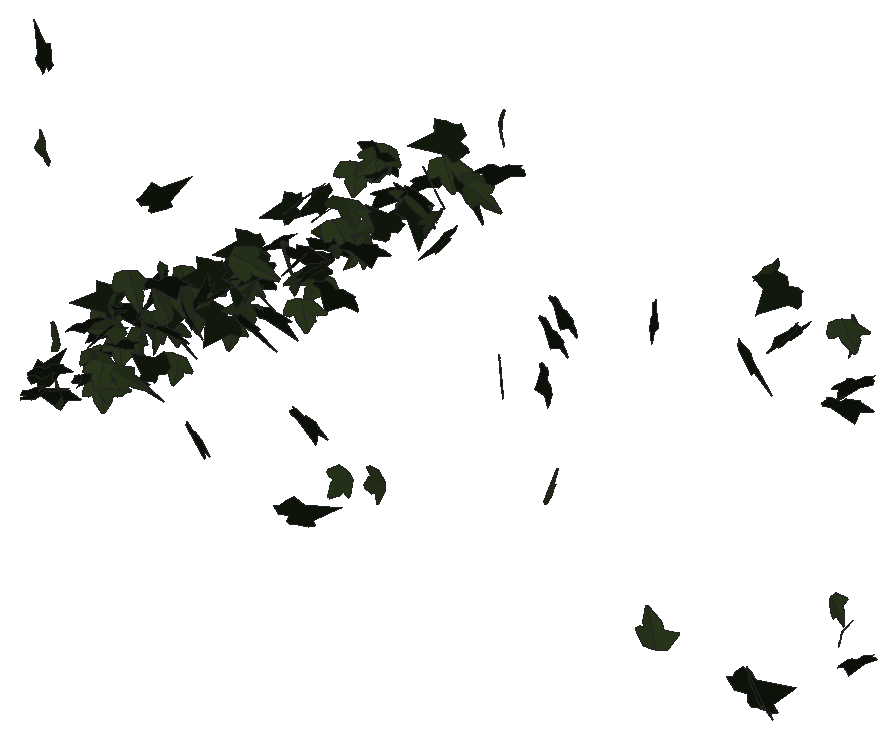
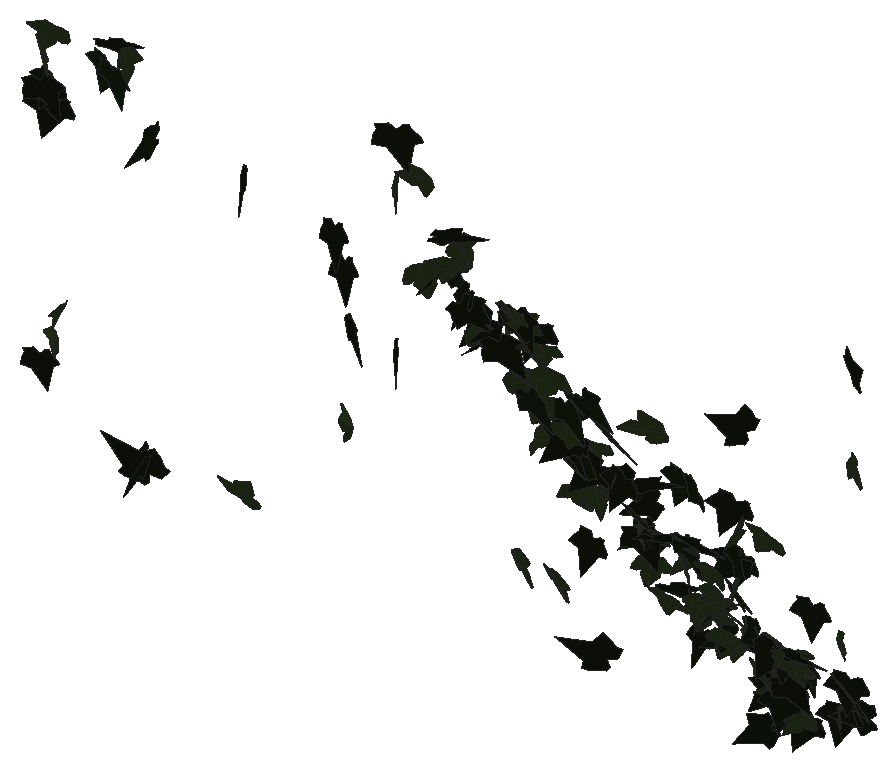
# SketchUp Ruby script. Lengths in inches.
U = 1.inch
M = Sketchup.active_model
def pt(a) = Geom::Point3d.new(a.map { |v| v * U })
def face(e, loops, mat)
  f = e.add_face(loops[0].map { |a| pt(a) })
  loops[1..].each { |l| e.add_face(l.map { |a| pt(a) }).erase! }
  f.material = f.back_material = mat if mat
  f
end
# faces: each face lists its corners as indices into pts; further lists are holes
def faces(e, pts, list, mat = nil) = list.each { |f| face(e, (f[0].is_a?(Array) ? f : [f]).map { |l| l.map { |i| pts[i] } }, mat) }
# xy, xz, yz: faces in a plane at the given z, y or x. An outline is a flat list of corners, or four numbers for a rectangle; further outlines are holes
def ring(l) = l.size == 4 ? [[l[0], l[1]], [l[2], l[1]], [l[2], l[3]], [l[0], l[3]]] : l.each_slice(2).to_a
def flat(e, list, mat, &to3) = list.each { |f| face(e, (f[0].is_a?(Array) ? f : [f]).map { |l| ring(l).map { |u, v| to3.(u, v) } }, mat) }
def xy(e, z, list, mat = nil) = flat(e, list, mat) { |x, y| [x, y, z] }
def xz(e, y, list, mat = nil) = flat(e, list, mat) { |x, z| [x, y, z] }
def yz(e, x, list, mat = nil) = flat(e, list, mat) { |y, z| [x, y, z] }
def lines(e, pts, list) = list.each { |a, b| e.add_line(pt(pts[a]), pt(pts[b])) }
# prism: a flat outline (further loops are holes) pulled along v
def prism(e, loops, v, mat = nil)
  f = face(e, loops, mat); d = Geom::Vector3d.new(v.map { |x| x * U })
  f.pushpull(f.normal.samedirection?(d) ? d.length : -d.length)
end
def box(e, o, s, mat = nil) = prism(e, [[o, [o[0] + s[0], o[1], o[2]], [o[0] + s[0], o[1] + s[1], o[2]], [o[0], o[1] + s[1], o[2]]]], [0, 0, s[2]], mat)
def at(x, y, z, deg = 0) = Geom::Transformation.translation(pt([x, y, z])) * Geom::Transformation.rotation(ORIGIN, Z_AXIS, deg.degrees)
def axes(o, x, y, z) = Geom::Transformation.new([*x, 0, *y, 0, *z, 0, *pt(o).to_a, 1])
def part(name) = M.definitions.add(name)
# library, detail: a bought-in or finely detailed component or shape, given as its bounding box
def library(name, o, s) = part(name).tap { |d| box(d.entities, o, s) }
def detail(e, o, s) = box(e.add_group.entities, o, s)
def put(e, d, t, mat = nil) = e.add_instance(d, t).tap { |i| i.material = mat if mat }
def group(e, t, mat = nil) = e.add_group.tap { |g| g.transformation = t; g.material = mat if mat }.entities
root = M.entities
M.materials.add("1026 AP 7946 SUNNY SIDE UP").color = [254, 231, 186]
M.materials.add("efeu1").color = [18, 25, 13]
M.materials.add("efeu2").color = [43, 57, 29]
c1 = part("ivyleaf_10")
p = [[0,0.5,-0.03],[-0.0625,2.02,-0.43],[-0.19,2.01,-0.46],[-0.54,1.05,-0.29],[-0.52,0.625,-0.18],[-0.83,0.76,-0.28],
  [-1.16,0.64,-0.33],[-1.15,0.33,-0.24],[-0.77,-0.39,0.02],[-0.3,-0.51,0.16],[0.04,-0.48,0.23],[-0.02,2.01,-0.4375],
  [-0.06,2.01,-0.43],[0.04,-0.49,0.23],[0.67,-0.49,0.14],[1.38,0.36,-0.2],[1.375,0.51,-0.24],[0.81,0.65,-0.19],
  [0.62,0.59,-0.15],[0.6,1.09,-0.28],[0.5,1.23,-0.31]]
faces(c1.entities,p,[[0,1,2,3,4,5,6,7,8,9,10],[11,12,0,13,14,15,16,17,18,19,20]],"efeu2")
c2 = part("ivyleaf_9")
p = [[1.54,2.16,1.25],[1.36,2.04,1.19],[-0.21,0.99,0.68],[-0.71,1.11,0.82],[-0.85,0.86,0.67],[-0.8,0.17,0.21],
  [-0.9,-0.01,0.1],[-0.67,-0.16,-0.02],[-0.08,-0.08,-0.05],[-0.03,-0.6,-0.4],[0.65,-0.88,-0.66],[0.83,-0.6,-0.49],
  [1.29,-0.42,-0.43],[1.8125,-0.07,-0.26],[1.21,0.44,0.15]]
faces(c2.entities,p,[[0,1,2,3,4,5,6,7,8,9,10,11,12,13,14]],"efeu1")
put(root,c1,axes([119.91,212.96,275.25],[-0.15786,0.09565,0.26441],[-0.34427,0.13528,-0.13967],[-0.25746,-0.23953,0.02464]),"1026 AP 7946 SUNNY SIDE UP")
put(root,c2,axes([119.46,212.93,268.7],[0.22563,0.03038,0.22502],[0.27226,0.14554,-0.1373],[-0.2143,0.21689,0.06248]),"1026 AP 7946 SUNNY SIDE UP")
put(root,c2,axes([119.64,213.11,269.07],[-0.17228,0.27616,0.11],[0.07778,-0.09348,0.30532],[0.45812,0.11972,-0.01047]),"1026 AP 7946 SUNNY SIDE UP")
put(root,c2,axes([119.96,212.91,277.56],[0.02395,-0.02649,0.33545],[-0.08757,0.32114,0.03146],[-0.50642,-0.05678,0.01042]),"1026 AP 7946 SUNNY SIDE UP")
put(root,c2,axes([119.96,212.98,269.53],[0.1913,0.22813,-0.05414],[-0.02362,-0.05296,-0.2664],[-0.36782,0.12205,-0.01105]),"1026 AP 7946 SUNNY SIDE UP")
put(root,c1,axes([120.09,213.29,268.71],[-0.01512,0.00573,-0.26968],[-0.14913,0.24412,0.01053],[0.38382,0.09508,-0.00654]),"1026 AP 7946 SUNNY SIDE UP")
put(root,c2,axes([119.97,213.21,268.81],[0.27016,0.18563,-0.0682],[-0.07693,-0.04634,-0.26081],[-0.30077,0.1786,0.00545]),"1026 AP 7946 SUNNY SIDE UP")
put(root,c1,axes([120.29,212.93,270.43],[-0.03129,-0.00435,-0.27853],[-0.17285,0.24779,0.00568],[0.38842,0.10992,-0.01991]),"1026 AP 7946 SUNNY SIDE UP")
put(root,c1,axes([120.02,214.64,269.24],[-0.20622,-0.18907,-0.13238],[0.24349,0.03403,-0.21602],[0.26314,-0.17967,0.09614]),"1026 AP 7946 SUNNY SIDE UP")
put(root,c1,axes([120.26,214.67,270.56],[0.41937,0.01395,-0.04707],[-0.06964,-0.02611,-0.27423],[-0.02847,0.26935,-0.02255]),"1026 AP 7946 SUNNY SIDE UP")
put(root,c2,axes([120.25,214.14,268.92],[0.27349,0.19928,-0.00399],[0.01534,-0.01514,-0.272],[-0.31307,0.17334,-0.01681]),"1026 AP 7946 SUNNY SIDE UP")
put(root,c2,axes([120.48,214.59,270.05],[0.01871,0.2119,-0.1617],[-0.10982,-0.15018,-0.21357],[-0.401,0.05102,0.05095]),"1026 AP 7946 SUNNY SIDE UP")
put(root,c2,axes([120.63,214.65,270.8],[-0.36738,0.02844,0.14169],[-0.21929,-0.01824,-0.24058],[-0.02385,-0.27042,0.02952]),"1026 AP 7946 SUNNY SIDE UP")
put(root,c1,axes([120.27,214.49,269.3],[-0.39403,0.07374,-0.08104],[0.10252,-0.05619,-0.26715],[-0.13563,-0.2567,0.0335]),"1026 AP 7946 SUNNY SIDE UP")
put(root,c2,axes([120.49,214.66,268.96],[-0.24093,-0.22018,0.04193],[-0.01299,-0.04524,-0.27593],[0.35221,-0.15229,0.01851]),"1026 AP 7946 SUNNY SIDE UP")
put(root,c2,axes([120.57,214.67,269.59],[0.15949,0.24453,-0.00867],[-0.00799,-0.00851,-0.27277],[-0.38472,0.10155,0.00207]),"1026 AP 7946 SUNNY SIDE UP")
put(root,c1,axes([120.8,214.41,270.27],[0.11431,0.06577,-0.26321],[-0.39441,-0.06612,-0.09131],[-0.13039,0.25765,0.04546]),"1026 AP 7946 SUNNY SIDE UP")
put(root,c1,axes([120.62,214.61,270.73],[-0.05219,0.21044,0.17672],[-0.07529,0.16435,-0.21782],[-0.41901,-0.05574,0.01713]),"1026 AP 7946 SUNNY SIDE UP")
put(root,c2,axes([120.75,214.37,270.31],[-0.17195,0.20293,-0.15062],[0.0715,-0.14205,-0.23712],[-0.3878,-0.11617,0.02307]),"1026 AP 7946 SUNNY SIDE UP")
put(root,c1,axes([120.7,213.97,268.87],[0.34189,0.14817,0.03738],[0.06074,0.00614,-0.27049],[-0.23172,0.22022,-0.01574]),"1026 AP 7946 SUNNY SIDE UP")
put(root,c1,axes([120.74,214.68,269.73],[0.32211,0.16897,-0.00307],[0.01634,-0.01878,-0.27281],[-0.26525,0.20403,-0.02054]),"1026 AP 7946 SUNNY SIDE UP")
put(root,c2,axes([120.79,214.58,269.77],[0.33822,0.14743,0.0544],[0.08034,0.01723,-0.26814],[-0.2323,0.22061,-0.01353]),"1026 AP 7946 SUNNY SIDE UP")
put(root,c2,axes([121.125,213.16,269.66],[-0.06173,0.24971,0.08639],[-0.03885,0.07948,-0.25967],[-0.41165,-0.04495,0.01155]),"1026 AP 7946 SUNNY SIDE UP")
put(root,c2,axes([120.89,214.5625,270.75],[0.32899,0.16773,-0.01701],[-0.00017,-0.02769,-0.27553],[-0.26517,0.20812,-0.02092]),"1026 AP 7946 SUNNY SIDE UP")
put(root,c2,axes([121.04,212.99,271.1],[0.10218,0.26159,0.00145],[-0.00734,0.00108,-0.27763],[-0.41125,0.06497,0.00531]),"1026 AP 7946 SUNNY SIDE UP")
put(root,c2,axes([120.8,214.875,268.82],[0.42122,-0.02405,0.03637],[0.05631,0.00262,-0.277],[0.03694,0.2702,0.00752]),"1026 AP 7946 SUNNY SIDE UP")
put(root,c1,axes([121.34,213.29,269.91],[0.35846,0.13176,-0.0463],[-0.04318,-0.04344,-0.27043],[-0.21499,0.22841,-0.02289]),"1026 AP 7946 SUNNY SIDE UP")
put(root,c1,axes([121.26,214.71,270.125],[0.31847,-0.13253,0.1168],[0.15104,-0.06165,-0.24971],[0.22982,0.22416,0.00225]),"1026 AP 7946 SUNNY SIDE UP")
put(root,c1,axes([121.31,213.47,269.3],[0.0223,-0.11422,-0.24883],[0.23509,0.20313,-0.08897],[0.34707,-0.13025,0.07625]),"1026 AP 7946 SUNNY SIDE UP")
put(root,c2,axes([121.5,214.43,270.85],[0.07705,0.0999,0.26153],[0.12751,0.24034,-0.1124],[-0.40872,0.09381,0.01424]),"1026 AP 7946 SUNNY SIDE UP")
put(root,c1,axes([121.67,214.7,270.68],[0.1666,0.25002,0.0705],[0.05344,0.05835,-0.27927],[-0.40349,0.11096,-0.00788]),"1026 AP 7946 SUNNY SIDE UP")
put(root,c1,axes([121.65,214.41,270.84],[-0.171,0.10534,-0.23901],[0.20783,-0.19309,-0.15487],[-0.34353,-0.16925,0.02528]),"1026 AP 7946 SUNNY SIDE UP")
put(root,c1,axes([121.88,214.58,270.57],[-0.01676,0.23894,-0.14875],[-0.01049,-0.14602,-0.24698],[-0.43996,-0.00562,0.01156]),"1026 AP 7946 SUNNY SIDE UP")
put(root,c1,axes([121.97,214.63,272.05],[-0.15017,0.25701,0.03144],[-0.03386,0.02297,-0.28205],[-0.40529,-0.09715,0.01191]),"1026 AP 7946 SUNNY SIDE UP")
put(root,c2,axes([122.11,214.61,271.91],[-0.33312,0.07759,-0.16813],[0.21896,-0.09123,-0.23082],[-0.18208,-0.25167,0.03003]),"1026 AP 7946 SUNNY SIDE UP")
put(root,c1,axes([121.8,213.35,269.86],[0.12396,0.00046,0.2645],[0.37022,0.10696,-0.07405],[-0.16098,0.24636,0.03337]),"1026 AP 7946 SUNNY SIDE UP")
put(root,c1,axes([122.17,214.77,270.69],[-0.42176,0.0219,-0.02374],[0.03258,-0.02942,-0.27596],[-0.03809,-0.26761,0.0268]),"1026 AP 7946 SUNNY SIDE UP")
put(root,c2,axes([122.09,214.71,270.67],[0.30629,-0.18532,0.01811],[0.03364,-0.00452,-0.27676],[0.29093,0.19563,0.01294]),"1026 AP 7946 SUNNY SIDE UP")
put(root,c2,axes([122.31,214.8,271.34],[-0.13753,-0.25693,0.08002],[-0.00879,-0.08146,-0.27931],[0.42264,-0.0853,0.02023]),"1026 AP 7946 SUNNY SIDE UP")
put(root,c1,axes([122.2,213.18,272.57],[0.44241,-0.00955,0.17236],[0.26066,-0.03276,-0.28922],[0.03918,0.32573,-0.02211]),"1026 AP 7946 SUNNY SIDE UP")
put(root,c1,axes([122.47,214.74,271.51],[0.40201,0.11508,-0.04344],[-0.05353,-0.02862,-0.28874],[-0.1855,0.25764,-0.01084]),"1026 AP 7946 SUNNY SIDE UP")
put(root,c2,axes([122.82,213.43,270.25],[-0.11045,0.18845,0.19054],[-0.22804,0.13115,-0.19478],[-0.34555,-0.14679,0.06763]),"1026 AP 7946 SUNNY SIDE UP")
put(root,c1,axes([122.54,214.7,271.67],[-0.37148,0.11771,-0.06832],[0.06243,-0.06857,-0.2688],[-0.2036,-0.23579,0.04223]),"1026 AP 7946 SUNNY SIDE UP")
put(root,c2,axes([122.64,214.67,271.32],[0.29862,-0.1524,-0.15109],[-0.20205,0.07196,-0.24951],[0.26297,0.22835,-0.02014]),"1026 AP 7946 SUNNY SIDE UP")
put(root,c1,axes([122.6,214.71,272.21],[-0.34287,0.01437,-0.17148],[0.20947,-0.1504,-0.19394],[-0.15876,-0.22948,0.11445]),"1026 AP 7946 SUNNY SIDE UP")
put(root,c1,axes([122.73,214.83,271.44],[-0.40714,-0.03692,-0.08263],[0.1291,-0.01102,-0.2686],[0.05025,-0.27078,0.02058]),"1026 AP 7946 SUNNY SIDE UP")
put(root,c1,axes([122.82,214.77,271.22],[-0.42227,-0.04463,-0.01242],[0.0236,-0.01854,-0.27975],[0.06865,-0.26817,0.01979]),"1026 AP 7946 SUNNY SIDE UP")
put(root,c2,axes([123.05,212.97,271.68],[0.09048,0.24156,0.12199],[0.01503,0.11778,-0.25458],[-0.4218,0.05601,0.0171]),"1026 AP 7946 SUNNY SIDE UP")
put(root,c1,axes([123.08,213.79,270.49],[0.41808,-0.04437,0.04911],[0.06811,-0.03056,-0.2769],[0.07686,0.26844,-0.02178]),"1026 AP 7946 SUNNY SIDE UP")
put(root,c1,axes([123.38,214.66,271.83],[0.17367,-0.06286,0.26351],[-0.28194,0.18575,0.1277],[-0.30413,-0.2081,0.03209]),"1026 AP 7946 SUNNY SIDE UP")
put(root,c1,axes([123.3,213.13,272.06],[-0.0832,0.32213,0.06446],[0.00305,-0.06122,0.33585],[0.51543,0.05236,0.00842]),"1026 AP 7946 SUNNY SIDE UP")
put(root,c2,axes([123.09,213.125,271.67],[0.41682,0.07036,0.00131],[-0.02005,0.05139,-0.27693],[-0.10882,0.26006,0.05606]),"1026 AP 7946 SUNNY SIDE UP")
put(root,c2,axes([123.0625,212.95,274.97],[0.02487,-0.02127,0.34048],[0.42124,0.19556,0.0009],[-0.30649,0.26705,0.02886]),"1026 AP 7946 SUNNY SIDE UP")
put(root,c2,axes([123.33,212.97,273.01],[0.29885,0.20143,-0.02348],[-0.00376,-0.03057,-0.2848],[-0.31893,0.18911,-0.01865]),"1026 AP 7946 SUNNY SIDE UP")
put(root,c2,axes([123.59,214.49,272.59],[-0.13453,0.27042,-0.02206],[-0.00194,-0.02445,-0.2922],[-0.42673,-0.08514,0.00828]),"1026 AP 7946 SUNNY SIDE UP")
put(root,c2,axes([123.75,214.53,272.57],[-0.39172,-0.0148,0.14308],[-0.21576,-0.02798,-0.25664],[0.04168,-0.28388,0.01615]),"1026 AP 7946 SUNNY SIDE UP")
put(root,c1,axes([123.38,214.48,272.24],[0.03253,0.15306,0.24681],[0.02599,0.23828,-0.15748],[-0.44512,0.0251,0.00884]),"1026 AP 7946 SUNNY SIDE UP")
put(root,c2,axes([123.77,214.74,271.45],[-0.34641,-0.17842,0.00937],[0.00524,-0.02014,-0.2916],[0.28095,-0.21962,0.01698]),"1026 AP 7946 SUNNY SIDE UP")
put(root,c1,axes([123.79,214.875,271.22],[0.43113,-0.03574,0.06445],[0.09194,-0.03478,-0.28377],[0.06666,0.27912,-0.02542]),"1026 AP 7946 SUNNY SIDE UP")
put(root,c2,axes([124.14,214.91,272.6875],[-0.25797,-0.22001,-0.05408],[0.0726,0.02935,-0.28187],[0.34771,-0.16936,0.01873]),"1026 AP 7946 SUNNY SIDE UP")
put(root,c2,axes([124.23,213.02,269.32],[0.33439,-0.05372,-0.18513],[-0.27803,0.03179,-0.22556],[0.09697,0.2764,-0.00834]),"1026 AP 7946 SUNNY SIDE UP")
put(root,c1,axes([124.35,214.74,271.88],[-0.35782,-0.17053,-0.03017],[0.06057,-0.00438,-0.2917],[0.26498,-0.22927,0.02593]),"1026 AP 7946 SUNNY SIDE UP")
put(root,c2,axes([124.51,214.85,272.62],[0.1352,0.21378,-0.16014],[-0.14804,-0.12931,-0.23579],[-0.38955,0.12334,0.03403]),"1026 AP 7946 SUNNY SIDE UP")
put(root,c2,axes([124.46,212.95,272.9],[0.08431,0.10245,0.26538],[0.01501,0.26096,-0.10769],[-0.4348,0.02887,0.04774]),"1026 AP 7946 SUNNY SIDE UP")
put(root,c1,axes([124.41,214.69,272.59],[0.43955,-0.01764,0.00607],[0.01103,0.0161,-0.28796],[0.02715,0.27914,0.01864]),"1026 AP 7946 SUNNY SIDE UP")
put(root,c1,axes([124.6,214.73,272.63],[0.07805,-0.28073,0.05767],[0.00356,-0.05805,-0.29392],[0.45059,0.04909,-0.00767]),"1026 AP 7946 SUNNY SIDE UP")
put(root,c2,axes([124.83,214.58,273.65],[-0.29029,-0.08435,0.2115],[-0.2663,-0.12003,-0.20791],[0.22666,-0.24904,0.02661]),"1026 AP 7946 SUNNY SIDE UP")
put(root,c2,axes([124.79,214.9375,273.13],[-0.40072,0.05865,-0.10457],[0.12632,-0.09055,-0.26136],[-0.13486,-0.25907,0.0659]),"1026 AP 7946 SUNNY SIDE UP")
put(root,c2,axes([124.46,214.73,272.62],[0.38559,-0.13239,-0.02917],[-0.04235,0.00813,-0.28699],[0.20837,0.24664,-0.00434]),"1026 AP 7946 SUNNY SIDE UP")
put(root,c2,axes([124.84,212.96,273.11],[0.11554,0.2327,0.14622],[-0.00659,0.14661,-0.24684],[-0.42747,0.06064,0.04333]),"1026 AP 7946 SUNNY SIDE UP")
put(root,c2,axes([125.08,214.83,273.79],[0.14241,0.24889,0.10151],[0.06735,0.0877,-0.27216],[-0.41466,0.09972,-0.00934]),"1026 AP 7946 SUNNY SIDE UP")
put(root,c1,axes([125.38,214.87,273.72],[-0.21498,0.25985,0.02267],[-0.02354,0.01532,-0.30234],[-0.40919,-0.1374,0.00548]),"1026 AP 7946 SUNNY SIDE UP")
put(root,c2,axes([125.68,214.85,274.94],[-0.3534,0.17955,0.01721],[-0.03674,-0.00416,-0.29581],[-0.28102,-0.22526,0.01702]),"1026 AP 7946 SUNNY SIDE UP")
put(root,c2,axes([125.32,213.4,272.53],[0.41497,-0.09215,0.03435],[0.03832,-0.03261,-0.28722],[0.14954,0.26407,-0.02173]),"1026 AP 7946 SUNNY SIDE UP")
put(root,c1,axes([125.8,214.89,273.21],[-0.03607,-0.29193,0.00067],[0.02434,-0.00353,-0.30126],[0.4584,-0.02279,0.01605]),"1026 AP 7946 SUNNY SIDE UP")
put(root,c1,axes([125.46,213.18,274.23],[0.11776,0.07495,0.33496],[0.47377,0.12699,-0.10104],[-0.22391,0.3081,-0.03763]),"1026 AP 7946 SUNNY SIDE UP")
put(root,c2,axes([126.11,214.77,273.95],[-0.23508,0.21845,-0.13365],[0.10324,-0.11368,-0.27321],[-0.38697,-0.16304,0.0083]),"1026 AP 7946 SUNNY SIDE UP")
put(root,c2,axes([125.84,214.82,273.88],[0.45183,0.06746,-0.00677],[0.00243,-0.03677,-0.302],[-0.1066,0.28507,-0.03557]),"1026 AP 7946 SUNNY SIDE UP")
put(root,c2,axes([126.22,214.84,275.53],[-0.21126,0.21167,-0.15144],[0.06281,-0.14801,-0.25596],[-0.40142,-0.13456,0.03965]),"1026 AP 7946 SUNNY SIDE UP")
put(root,c2,axes([125.93,213.49,272.89],[0.44526,0.0157,0.01005],[0.01733,-0.02483,-0.29114],[-0.02324,0.28225,-0.02451]),"1026 AP 7946 SUNNY SIDE UP")
put(root,c1,axes([126.33,214.98,273.21],[0.33236,0.17094,-0.11175],[-0.17432,-0.03513,-0.27731],[-0.26735,0.23542,0.04189]),"1026 AP 7946 SUNNY SIDE UP")
put(root,c2,axes([126.61,214.84,273.72],[-0.37626,0.17143,0.00407],[-0.03607,-0.02693,-0.30122],[-0.26718,-0.23778,0.03493]),"1026 AP 7946 SUNNY SIDE UP")
put(root,c2,axes([126.57,214.89,275.48],[-0.38443,0.13675,-0.07421],[0.07012,-0.06816,-0.28653],[-0.2333,-0.24583,0.03617]),"1026 AP 7946 SUNNY SIDE UP")
put(root,c2,axes([126.67,214.92,275.21],[-0.10874,0.27819,-0.03205],[-0.00152,-0.03391,-0.29536],[-0.44043,-0.06856,0.00894]),"1026 AP 7946 SUNNY SIDE UP")
put(root,c2,axes([126.69,214.3,273.81],[-0.02688,0.27633,0.08488],[-0.04486,0.07894,-0.2838],[-0.45048,-0.02435,0.0232]),"1026 AP 7946 SUNNY SIDE UP")
put(root,c1,axes([126.7,214.93,274.5625],[-0.45131,-0.00524,-0.02185],[0.03389,-0.0247,-0.29475],[0.00534,-0.28674,0.0241]),"1026 AP 7946 SUNNY SIDE UP")
put(root,c2,axes([126.55,214.82,274.4],[0.39352,0.15175,0.05785],[0.09503,0.00658,-0.30035],[-0.23551,0.25621,-0.02453]),"1026 AP 7946 SUNNY SIDE UP")
put(root,c2,axes([126.78,213.4,267.92],[0.0896,-0.01037,0.3133],[0.47539,0.03751,-0.05681],[-0.05503,0.30718,0.01934]),"1026 AP 7946 SUNNY SIDE UP")
put(root,c1,axes([127,213.48,273.43],[0.37612,0.15335,0.04751],[0.07068,0.01364,-0.29235],[-0.24127,0.24306,-0.01158]),"1026 AP 7946 SUNNY SIDE UP")
put(root,c1,axes([127.01,214.71,274.95],[0.35632,0.07186,0.18566],[0.28319,0.02348,-0.24335],[-0.11187,0.28833,-0.02466]),"1026 AP 7946 SUNNY SIDE UP")
put(root,c1,axes([127.33,215.1875,274.27],[0.02739,0.14947,-0.26415],[-0.11789,-0.24718,-0.15462],[-0.45273,0.07341,0.02428]),"1026 AP 7946 SUNNY SIDE UP")
put(root,c2,axes([127.3,213.2,270.73],[0.39369,0.00053,-0.16093],[-0.24515,-0.01793,-0.25758],[-0.01562,0.29457,-0.01366]),"1026 AP 7946 SUNNY SIDE UP")
put(root,c1,axes([127.3125,214.7,275.68],[-0.45218,-0.04498,-0.06702],[0.10848,-0.02468,-0.29792],[0.06012,-0.29375,0.03352]),"1026 AP 7946 SUNNY SIDE UP")
put(root,c1,axes([127.38,214.95,276.49],[0.41861,0.13077,0.00118],[0.01822,-0.02268,-0.30457],[-0.20481,0.26526,-0.02468]),"1026 AP 7946 SUNNY SIDE UP")
put(root,c2,axes([127.71,214.98,275.17],[-0.14104,0.27092,-0.05738],[-0.03546,-0.06711,-0.29125],[-0.43396,-0.08257,0.04245]),"1026 AP 7946 SUNNY SIDE UP")
put(root,c1,axes([127.68,214.89,274.78],[0.34972,-0.14242,0.14624],[0.18429,-0.08167,-0.27251],[0.25804,0.25135,-0.00358]),"1026 AP 7946 SUNNY SIDE UP")
put(root,c2,axes([127.95,213.53,274.14],[0.28719,0.07705,-0.21966],[-0.28801,-0.11216,-0.20363],[-0.21119,0.25774,-0.02102]),"1026 AP 7946 SUNNY SIDE UP")
put(root,c1,axes([127.98,215.01,277.01],[0.23041,0.15928,-0.21331],[-0.22181,-0.1528,-0.22386],[-0.34706,0.2034,0.00146]),"1026 AP 7946 SUNNY SIDE UP")
put(root,c2,axes([128.09,214.97,277.16],[0.25457,0.0366,-0.25737],[-0.35796,-0.10779,-0.16874],[-0.1725,0.27769,-0.02968]),"1026 AP 7946 SUNNY SIDE UP")
put(root,c1,axes([128.14,214.89,275.45],[-0.24493,-0.13764,0.22792],[-0.18215,-0.19529,-0.2096],[0.36815,-0.1882,0.04793]),"1026 AP 7946 SUNNY SIDE UP")
put(root,c2,axes([128.36,214.88,276.92],[-0.246,0.25138,-0.01503],[-0.01137,-0.02333,-0.30457],[-0.39591,-0.15553,0.01808]),"1026 AP 7946 SUNNY SIDE UP")
put(root,c1,axes([128.21,215.03,277.19],[0.44295,-0.09701,0.0437],[0.05236,-0.03492,-0.3063],[0.1584,0.28281,-0.02095]),"1026 AP 7946 SUNNY SIDE UP")
put(root,c1,axes([128.37,213.28,269.51],[0.38788,-0.18782,-0.06635],[-0.09912,0.02153,-0.31857],[0.29549,0.25377,-0.01977]),"1026 AP 7946 SUNNY SIDE UP")
put(root,c2,axes([128.54,215.02,276.26],[0.01317,0.21705,-0.20364],[-0.09718,-0.19326,-0.22106],[-0.45261,0.04781,0.04154]),"1026 AP 7946 SUNNY SIDE UP")
put(root,c2,axes([128.82,214.41,275.63],[-0.07705,0.16835,0.24677],[-0.22603,0.19667,-0.17223],[-0.39965,-0.14369,0.04983]),"1026 AP 7946 SUNNY SIDE UP")
put(root,c2,axes([128.9,213.21,275.78],[0.35776,0.17047,-0.07718],[-0.08619,-0.05333,-0.29304],[-0.28046,0.23384,-0.0084]),"1026 AP 7946 SUNNY SIDE UP")
put(root,c1,axes([129.16,214.94,276.27],[-0.39418,-0.08339,0.16236],[-0.18762,-0.12463,-0.26341],[0.20922,-0.26888,0.06968]),"1026 AP 7946 SUNNY SIDE UP")
put(root,c1,axes([129.32,213.39,269.67],[0.23268,-0.17022,-0.23405],[-0.22672,0.17436,-0.2313],[0.3831,0.20657,0.00527]),"1026 AP 7946 SUNNY SIDE UP")
put(root,c2,axes([129.02,214.8,276.57],[0.4765,-0.01101,-0.03765],[-0.05864,-0.02546,-0.31134],[0.01234,0.30416,-0.02563]),"1026 AP 7946 SUNNY SIDE UP")
put(root,c2,axes([129.15,214.99,276.02],[-0.02567,-0.30008,0.05815],[-0.00772,-0.05796,-0.30993],[0.48057,-0.01696,-0.00187]),"1026 AP 7946 SUNNY SIDE UP")
put(root,c2,axes([129.53,215.11,276.95],[-0.11832,0.17298,-0.23662],[-0.01092,-0.23941,-0.18402],[-0.45322,-0.03939,0.06621]),"1026 AP 7946 SUNNY SIDE UP")
put(root,c2,axes([129.65,214.83,277.07],[0.34181,-0.10433,-0.19749],[-0.28103,0.06874,-0.24769],[0.19555,0.28116,-0.01076]),"1026 AP 7946 SUNNY SIDE UP")
put(root,c1,axes([129.81,214.99,278.16],[-0.33666,0.21171,0.00656],[-0.02897,-0.0113,-0.3095],[-0.33173,-0.21387,0.02037]),"1026 AP 7946 SUNNY SIDE UP")
put(root,c2,axes([130.42,214.88,278.3125],[-0.32563,-0.07483,0.22339],[-0.29108,-0.11895,-0.22468],[0.21407,-0.27557,0.03429]),"1026 AP 7946 SUNNY SIDE UP")
put(root,c1,axes([130.16,214.76,277.66],[0.34451,0.20908,0.06606],[0.08507,0.03439,-0.31154],[-0.33263,0.22535,-0.01126]),"1026 AP 7946 SUNNY SIDE UP")
put(root,c1,axes([130.81,215.08,277.36],[-0.34908,-0.20597,0.07706],[-0.0341,-0.08694,-0.30862],[0.34351,-0.21794,0.04767]),"1026 AP 7946 SUNNY SIDE UP")
put(root,c2,axes([130.51,215.01,277.23],[0.18201,-0.28498,0.05097],[0.01639,-0.05089,-0.31703],[0.45496,0.11584,-0.00897]),"1026 AP 7946 SUNNY SIDE UP")
put(root,c1,axes([131,213.35,277.27],[-0.01284,-0.29505,0.06113],[0.00011,-0.06104,-0.30443],[0.47376,-0.00799,0.00173]),"1026 AP 7946 SUNNY SIDE UP")
put(root,c2,axes([131.21,213.55,276.64],[-0.28986,0.21399,-0.10859],[0.07307,-0.09999,-0.29011],[-0.36877,-0.18802,0.02787]),"1026 AP 7946 SUNNY SIDE UP")
put(root,c1,axes([131.76,214.81,279.21],[-0.15483,0.21656,0.21283],[-0.24503,0.14712,-0.23595],[-0.40023,-0.17385,0.06212]),"1026 AP 7946 SUNNY SIDE UP")
put(root,c1,axes([132.28,213.18,278.45],[-0.21044,-0.01817,-0.28165],[0.39575,-0.12815,-0.11895],[-0.1699,-0.276,0.0718]),"1026 AP 7946 SUNNY SIDE UP")
put(root,c2,axes([132.93,213.32,273.87],[0.14312,-0.06053,-0.30502],[-0.41989,0.12789,-0.11089],[0.22133,0.28176,-0.01313]),"1026 AP 7946 SUNNY SIDE UP")
put(root,c2,axes([133.1,213.09,279.34],[0.13775,0.25753,-0.14705],[-0.08278,-0.13437,-0.28096],[-0.45665,0.10204,0.00657]),"1026 AP 7946 SUNNY SIDE UP")
put(root,c2,axes([134.24,213.37,274.0625],[0.09177,-0.04555,-0.32115],[-0.47753,0.07522,-0.06952],[0.13027,0.30784,-0.02859]),"1026 AP 7946 SUNNY SIDE UP")
put(root,c2,axes([134.47,213.28,275.49],[0.28223,-0.00649,-0.27279],[-0.41409,0.02952,-0.18449],[0.04412,0.3185,0.01342]),"1026 AP 7946 SUNNY SIDE UP")
put(root,c1,axes([134.4375,213.1875,271.21],[0.1932,-0.18132,0.23886],[-0.16266,0.20981,0.22574],[-0.43466,-0.15911,0.02169]),"1026 AP 7946 SUNNY SIDE UP")
put(root,c2,axes([134.85,213.17,276.22],[0.28955,-0.02352,-0.26993],[-0.41059,0.02117,-0.19099],[0.04852,0.31945,-0.00533]),"1026 AP 7946 SUNNY SIDE UP")
put(root,c2,axes([137.35,213.35,276.85],[0.09883,-0.0668,-0.32682],[-0.40866,0.18214,-0.09161],[0.30375,0.26679,-0.01691]),"1026 AP 7946 SUNNY SIDE UP")
put(root,c1,axes([137.43,213.34,268.41],[0.50252,-0.00727,0.14514],[-0.21675,0.05857,0.3255],[-0.04748,-0.34434,0.05022]),"1026 AP 7946 SUNNY SIDE UP")
put(root,c2,axes([139.97,213.38,276.85],[0.4002,-0.22549,-0.11426],[-0.15009,0.0573,-0.3494],[0.36455,0.27113,-0.01842]),"1026 AP 7946 SUNNY SIDE UP")
put(root,c2,axes([140.28,213.3,268.38],[0.3789,-0.18087,-0.20271],[-0.27927,0.08778,-0.30828],[0.31246,0.29779,-0.02971]),"1026 AP 7946 SUNNY SIDE UP")
put(root,c1,axes([140.46,213.76,279.03],[-0.05655,-0.29597,-0.04192],[0.03144,0.03682,-0.30653],[0.46835,-0.0382,0.01551]),"1026 AP 7946 SUNNY SIDE UP")
put(root,c2,axes([140.21,213.29,268.02],[-0.03161,0.01696,0.3689],[0.4808,-0.18621,0.02569],[0.29395,0.30641,-0.00235]),"1026 AP 7946 SUNNY SIDE UP")
put(root,c2,axes([141.21,213.38,278.96],[-0.42371,-0.13572,0.01766],[-0.01039,-0.0266,-0.31024],[0.215,-0.26875,0.01981]),"1026 AP 7946 SUNNY SIDE UP")
put(root,c2,axes([141.49,212.93,277.88],[-0.06885,0.29126,0.10989],[-0.01494,0.10475,-0.30276],[-0.48661,-0.04443,-0.00625]),"1026 AP 7946 SUNNY SIDE UP")
put(root,c2,axes([141.68,212.92,277.97],[0.09526,0.23398,0.2053],[-0.01426,0.20306,-0.24322],[-0.4817,0.04026,0.0478]),"1026 AP 7946 SUNNY SIDE UP")
put(root,c1,axes([142.99,213.23,270.56],[0.06625,0.12987,0.23314],[-0.25051,0.19357,-0.08303],[-0.32365,-0.12324,0.11198]),"1026 AP 7946 SUNNY SIDE UP")
put(root,c1,axes([142.8125,213.16,271.36],[-0.04149,0.26897,0.05365],[-0.00055,0.05075,-0.27809],[-0.43034,-0.026,-0.00482]),"1026 AP 7946 SUNNY SIDE UP")
put(root,c1,axes([143.12,213.53,278.3125],[0.10864,-0.20669,-0.30548],[-0.16818,0.27544,-0.22274],[0.54132,0.12706,-0.00789]),"1026 AP 7946 SUNNY SIDE UP")
put(root,c2,axes([143.02,213.18,276.67],[0.3431,0.17938,-0.0726],[-0.07682,-0.05309,-0.29114],[-0.29376,0.22339,-0.00866]),"1026 AP 7946 SUNNY SIDE UP")
put(root,c2,axes([143.23,213.39,277.2],[0.01174,0.25697,-0.15158],[-0.02202,-0.14818,-0.26556],[-0.46623,0.01347,0.00873]),"1026 AP 7946 SUNNY SIDE UP")
put(root,c1,axes([142.99,213.27,278.6],[0.40872,0.10454,0.11131],[0.13057,0.07868,-0.28532],[-0.19627,0.27004,0.04199]),"1026 AP 7946 SUNNY SIDE UP")
put(root,c2,axes([143.21,212.97,277],[0.157,0.22794,0.17655],[0.03708,0.173,-0.25211],[-0.44566,0.09469,0.04122]),"1026 AP 7946 SUNNY SIDE UP")
put(root,c2,axes([143.35,213.3,269.99],[0.05757,0.24525,-0.0759],[-0.0125,-0.0747,-0.25588],[-0.4031,0.03734,-0.00291]),"1026 AP 7946 SUNNY SIDE UP")
